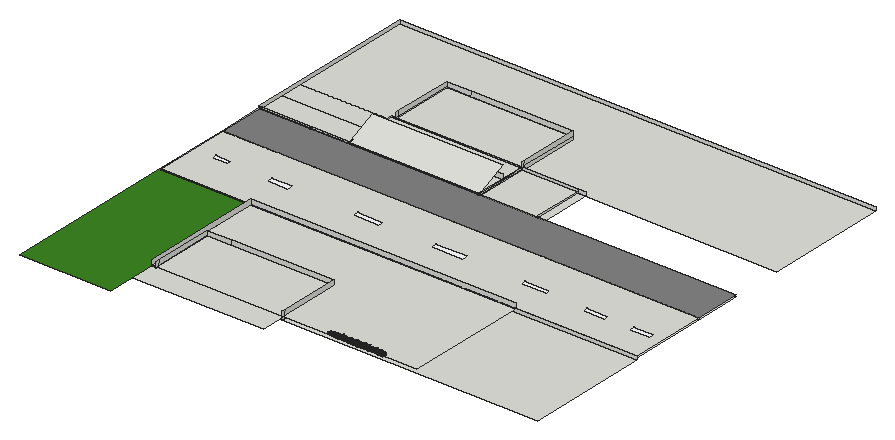
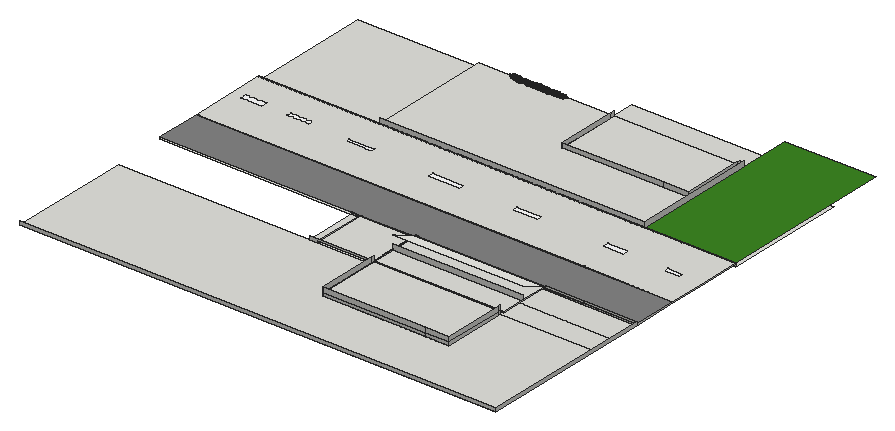
# SketchUp Ruby script. Lengths in inches.
U = 1.inch
M = Sketchup.active_model
def pt(a) = Geom::Point3d.new(a.map { |v| v * U })
def face(e, loops, mat)
  f = e.add_face(loops[0].map { |a| pt(a) })
  loops[1..].each { |l| e.add_face(l.map { |a| pt(a) }).erase! }
  f.material = f.back_material = mat if mat
  f
end
# faces: each face lists its corners as indices into pts; further lists are holes
def faces(e, pts, list, mat = nil) = list.each { |f| face(e, (f[0].is_a?(Array) ? f : [f]).map { |l| l.map { |i| pts[i] } }, mat) }
# xy, xz, yz: faces in a plane at the given z, y or x. An outline is a flat list of corners, or four numbers for a rectangle; further outlines are holes
def ring(l) = l.size == 4 ? [[l[0], l[1]], [l[2], l[1]], [l[2], l[3]], [l[0], l[3]]] : l.each_slice(2).to_a
def flat(e, list, mat, &to3) = list.each { |f| face(e, (f[0].is_a?(Array) ? f : [f]).map { |l| ring(l).map { |u, v| to3.(u, v) } }, mat) }
def xy(e, z, list, mat = nil) = flat(e, list, mat) { |x, y| [x, y, z] }
def xz(e, y, list, mat = nil) = flat(e, list, mat) { |x, z| [x, y, z] }
def yz(e, x, list, mat = nil) = flat(e, list, mat) { |y, z| [x, y, z] }
def lines(e, pts, list) = list.each { |a, b| e.add_line(pt(pts[a]), pt(pts[b])) }
# prism: a flat outline (further loops are holes) pulled along v
def prism(e, loops, v, mat = nil)
  f = face(e, loops, mat); d = Geom::Vector3d.new(v.map { |x| x * U })
  f.pushpull(f.normal.samedirection?(d) ? d.length : -d.length)
end
def box(e, o, s, mat = nil) = prism(e, [[o, [o[0] + s[0], o[1], o[2]], [o[0] + s[0], o[1] + s[1], o[2]], [o[0], o[1] + s[1], o[2]]]], [0, 0, s[2]], mat)
def at(x, y, z, deg = 0) = Geom::Transformation.translation(pt([x, y, z])) * Geom::Transformation.rotation(ORIGIN, Z_AXIS, deg.degrees)
def axes(o, x, y, z) = Geom::Transformation.new([*x, 0, *y, 0, *z, 0, *pt(o).to_a, 1])
def part(name) = M.definitions.add(name)
# library, detail: a bought-in or finely detailed component or shape, given as its bounding box
def library(name, o, s) = part(name).tap { |d| box(d.entities, o, s) }
def detail(e, o, s) = box(e.add_group.entities, o, s)
def put(e, d, t, mat = nil) = e.add_instance(d, t).tap { |i| i.material = mat if mat }
def group(e, t, mat = nil) = e.add_group.tap { |g| g.transformation = t; g.material = mat if mat }.entities
root = M.entities
M.materials.add("Color_3").color = [255, 255, 255]
M.materials.add("Material82").color = [68, 110, 58]
M.materials.add("Material83").color = [48, 90, 38]
M.materials.add("Material84").color = [68, 110, 48]
M.materials.add("Material85").color = [48, 90, 48]
M.materials.add("Material86").color = [58, 110, 58]
M.materials.add("Material87").color = [58, 90, 38]
M.materials.add("Material88").color = [68, 100, 58]
M.materials.add("Material89").color = [48, 100, 38]
M.materials.add("[Color M01]").color = [60, 133, 34]
M.materials.add("[Tile Grey]1").color = [132, 132, 132]
c1 = part("grass00")
p = [[-0.6875,0.15,0],[-0.56,0.08,5.52],[-0.04,0.03,2.76],[0.48,-0.02,0],[0.35,-0.02,5.52],[-0.1,-0.14,5.52],
  [-0.12,0.65,8.37],[-0.42,0.65,8.37]]
faces(c1.entities,p,[[0,1,2,3],[3,2,4],[1,5,2],[5,4,2],[1,6,5],[4,5,6],[7,6,1]])
c2 = part("Group16\#1")
put(c2.entities,c1,axes([1.44,-0.61,-0.01],[0.05352,0.12609,0],[-0.10704,0.04543,0.07239],[0.06664,-0.02828,0.11628]),"Material85")
put(c2.entities,c1,axes([0.76,-0.15,-0.01],[0.04676,0.24062,0],[-0.23162,0.04501,0.06642],[0.0652,-0.01267,0.23595]),"Material82")
put(c2.entities,c1,axes([0.79,0.01,-0.01],[-0.00606,0.34651,0],[-0.34381,-0.00602,0.0432],[0.04319,0.00076,0.34386]))
put(c2.entities,c1,axes([1,0.23,-0.01],[-0.07192,0.31144,0],[-0.28722,-0.06632,0.1236],[0.12043,0.02781,0.29478]),"Material84")
put(c2.entities,c1,axes([1.66,0.77,-0.01],[-0.13828,0.29651,0],[-0.21551,-0.1005,0.22471],[0.20365,0.09498,0.23779]),"Material89")
put(c2.entities,c1,axes([0.6875,0.52,-0.01],[-0.18126,0.24051,0],[-0.22746,-0.17142,0.09788],[0.07817,0.05891,0.28481]),"Material84")
put(c2.entities,c1,axes([0.68,0.78,-0.01],[-0.215,0.18688,0],[-0.12385,-0.14248,0.21334],[0.13995,0.16101,0.18878]),"Material82")
put(c2.entities,c1,axes([0.56,1,-0.01],[-0.13756,0.07624,0],[-0.06159,-0.11112,0.0927],[0.04494,0.08108,0.12705]),"Material84")
put(c2.entities,c1,axes([0.2,0.64,-0.01],[-0.23729,0.07254,0],[-0.05711,-0.18681,0.153],[0.04473,0.14632,0.19535]),"Material89")
put(c2.entities,c1,axes([0.0625,0.72,-0.01],[-0.28874,0.02525,0],[-0.02179,-0.24916,0.14647],[0.01276,0.14591,0.25012]),"Material82")
put(c2.entities,c1,axes([-0.08,0.62,-0.01],[-0.34089,-0.04187,0],[0.03255,-0.26504,0.216],[-0.02633,0.21439,0.26703]),"Material89")
put(c2.entities,c1,axes([-0.34,0.98,-0.01],[-0.14314,-0.0493,0],[0.04397,-0.12769,0.06843],[-0.02228,0.0647,0.13505]),"Material89")
put(c2.entities,c1,axes([-0.87,1.45,-0.01],[-0.23488,-0.14114,0],[0.13761,-0.22901,0.06087],[-0.03135,0.05217,0.26717]))
put(c2.entities,c1,axes([-0.72,0.77,-0.01],[-0.14208,-0.13251,0],[0.07209,-0.0773,0.16301],[-0.11118,0.11922,0.1057]),"Material89")
put(c2.entities,c1,axes([-0.62,0.43,-0.01],[-0.14845,-0.21203,0],[0.18654,-0.13061,0.12304],[-0.10079,0.07057,0.22772]),"Material82")
put(c2.entities,c1,axes([-0.68,0.29,-0.01],[-0.13639,-0.32136,0],[0.31723,-0.13464,0.05579],[-0.05136,0.0218,0.34462]),"Material83")
put(c2.entities,c1,axes([-0.64,0.125,-0.01],[-0.0458,-0.23569,0],[0.22124,-0.043,0.08276],[-0.08124,0.01579,0.22538]),"Material86")
put(c2.entities,c1,axes([-1.6,-0.03,-0.01],[0.00576,-0.32897,0],[0.27526,0.00482,0.18018],[-0.18015,-0.00315,0.2753]),"Material84")
put(c2.entities,c1,axes([-1.36,-0.31,-0.01],[0.05718,-0.24765,0],[0.18172,0.04196,0.17267],[-0.16825,-0.03885,0.1865]),"Material89")
put(c2.entities,c1,axes([-1.54,-0.72,-0.01],[0.06537,-0.14017,0],[0.13555,0.06321,0.03939],[-0.0357,-0.01665,0.14956]))
put(c2.entities,c1,axes([-1.19,-0.9,-0.01],[0.09597,-0.12735,0],[0.11214,0.08451,0.07557],[-0.06035,-0.04548,0.14042]),"Material88")
put(c2.entities,c1,axes([-0.47,-0.54,-0.01],[0.11588,-0.10072,0],[0.0618,0.0711,0.12124],[-0.07953,-0.0915,0.0942]))
put(c2.entities,c1,axes([-0.47,-0.84,-0.01],[0.11927,-0.0661,0],[0.06603,0.11913,0.00646],[-0.00313,-0.00565,0.13621]),"Material84")
put(c2.entities,c1,axes([-0.38,-1.24,-0.01],[0.28037,-0.08571,0],[0.0618,0.20215,0.20315],[-0.05939,-0.19428,0.21139]),"Material88")
put(c2.entities,c1,axes([-0.06,-0.66,-0.01],[0.22719,-0.01987,0],[0.01247,0.14255,0.17758],[-0.01547,-0.17691,0.1431]),"Material87")
put(c2.entities,c1,axes([0.11,-0.89,-0.01],[0.14882,0.01828,0],[-0.01058,0.08611,0.12229],[0.01491,-0.12138,0.08676]),"Material85")
put(c2.entities,c1,axes([0.25,-0.72,-0.01],[0.20481,0.07053,0],[-0.06206,0.18022,0.10291],[0.03351,-0.0973,0.1906]),"Material85")
put(c2.entities,c1,axes([0.85,-1.42,-0.01],[0.16481,0.09904,0],[-0.09472,0.15762,0.05616],[0.02893,-0.04814,0.18389]),"Material84")
put(c2.entities,c1,axes([1.01,-1.09,-0.01],[0.21858,0.20385,0],[-0.17495,0.1876,0.15339],[0.10462,-0.11218,0.25652]),"Material89")
put(c2.entities,c1,axes([1.01,-0.71,-0.01],[0.08733,0.12473,0],[-0.06445,0.04512,0.13037],[0.1068,-0.07477,0.07867]),"Material85")
c3 = part("Group15\#1")
put(c3.entities,c2,at(0,0,0))
c4 = part("3darcstudiotree_grass00\#1")
put(c4.entities,c3,at(0,0,0))
c5 = part("Untitled (5)")
xy(c5.entities,0,[[[158.81,26.5625,306.06,993.3125],[226.57,518.17,239.57,583.92],[225.28,357.51,237.28,411.51],[222.61,182.28,236.36,226.53],[239.71,931.55,251.46,972.3],[233.64,703.93,242.14,755.18],[240.05,835.03,248.8,880.53],[222.04,66.5,231.29,100.5]]])
xy(c5.entities,0,[[222.04,66.5,231.29,100.5],[222.61,182.28,236.36,226.53],[225.28,357.51,237.28,411.51],[226.57,518.17,239.57,583.92],[233.64,703.93,242.14,755.18],
  [240.05,835.03,248.8,880.53],[239.71,931.55,251.46,972.3]],"Color_3")
xy(root,-42.1875,[[0.34,387.84,0.34,659.09,1048.66,659.09,1048.66,387.84,486.41,387.84,486.41,528.53,208.91,528.53,208.91,387.84],[208.91,387.84,486.41,528.53]])
xy(root,-37.75,[[0,660.69,1048.3125,831.37],[0,831.37,199.6875,932.5],[199.6875,831.37,199.6875,932.5,486.07,932.5,486.07,1046.93,608.75,1046.93,608.75,932.5,1048.3125,932.5,1048.3125,831.37],[0,932.5,486.07,994.94],[608.75,932.5,626.34,1046.93],
  [0,994.94,486.07,1046.93],[0,1046.93,0,1318.18,1048.3125,1318.18,1048.3125,1046.93,486.07,1046.93,486.07,1187.62,208.57,1187.62,208.57,1046.93],[208.57,1046.93,486.07,1187.62]])
xy(root,-35.625,[[200.03,335.84,486.41,335.84,486.41,528.53,208.91,528.53,208.91,387.84,200.03,387.84]])
xy(root,-34.75,[[0,660.69,1048.3125,831.37]])
xy(root,-34.6875,[[486.07,932.5,608.75,1046.93]])
xy(root,-34.17,[[200.03,387.84,782.78,659.09]])
xy(root,-34.17,[[0.34,273.53,200.03,659.09]],"[Color M01]")
xy(root,-34.17,[[0,831.37,1048.3125,932.5]],"[Tile Grey]1")
xy(root,-33.625,[[0,932.5,115.625,932.62],[115.625,932.5,486.07,932.62]])
xy(root,-31.1875,[[199.6875,932.5,486.07,932.62],[199.6875,932.62,486.07,994.94],[199.6875,994.94,486.07,994.94,486.07,1187.62,208.57,1187.62,208.57,1046.93,199.6875,1046.93]])
xz(root,528.53,[[208.91,-42.1875,262.79,-35.625],[262.79,-42.1875,486.41,-35.625],[208.91,-35.625,262.79,-24.25],[262.79,-35.625,486.41,-24.25]])
xz(root,659.09,[[0.34,-42.1875,1048.66,-34.17],[200.03,-34.17,782.78,-22.8]])
xz(root,660.69,[[0,-37.75,1048.3125,-34.75]])
xz(root,831.37,[[0,-37.75,199.6875,-34.75],[199.6875,-37.75,1048.3125,-34.75],[0,-34.75,199.6875,-34.17],[199.6875,-34.75,1048.3125,-34.17]])
xz(root,932.5,[[0,-37.75,199.6875,-34.17],[199.6875,-37.75,486.07,-34.6875],[608.75,-37.75,626.34,-34.6875],[199.6875,-34.6875,486.07,-34.17],[486.07,-34.6875,608.75,-34.17],
  [608.75,-34.6875,626.34,-34.17],[0,-34.17,486.07,-33.75],[486.07,-34.17,608.75,-33.75],[608.75,-34.17,626.34,-33.75],[0,-33.75,486.07,-33.625],
  [115.625,-33.625,486.07,-33.625,486.07,-31.1875,199.6875,-31.1875,199.6875,-29.74,115.625,-29.74]])
xz(root,932.62,[[0,-33.625,115.625,-29.74],[115.625,-33.625,115.625,-29.74,199.6875,-29.74,199.6875,-31.1875,486.07,-31.1875,486.07,-33.625]])
xz(root,994.94,[[199.6875,-31.1875,486.07,-19.8125]])
xz(root,1046.93,[[208.57,-37.75,486.07,-29.74],[608.75,-37.75,626.34,-29.74],[486.07,-34.6875,608.75,-29.74],[199.6875,-31.1875,208.57,-29.74]])
xz(root,1187.62,[[208.57,-37.75,262.44,-31.1875],[262.44,-37.75,486.07,-31.1875],[208.57,-31.1875,262.44,-19.8125],[262.44,-31.1875,486.07,-19.8125]])
xz(root,1318.18,[[0,-37.75,1048.3125,-29.74]])
yz(root,0,[[660.69,-37.75,750.06,-34.75],[750.06,-37.75,831.37,-34.75],[831.37,-37.75,932.5,-34.17],[932.5,-37.75,932.5,-33.625,932.62,-33.625,932.62,-29.74,1318.18,-29.74,1318.18,-37.75]])
yz(root,115.625,[[932.5,-33.625,932.62,-29.74]])
yz(root,199.6875,[[932.5,-31.1875,932.62,-31.13,932.62,-29.74,932.5,-29.74],[932.5,-31.1875,932.62,-31.1875,932.62,-31.13],[932.62,-31.1875,932.62,-31.13,935.62,-29.74,994.94,-29.74,994.94,-31.1875],[994.94,-31.1875,1046.93,-29.74],[932.62,-31.13,935.62,-29.74,932.62,-29.74]])
yz(root,200.03,[[387.84,-34.17,659.09,-22.8]])
yz(root,208.57,[[1046.93,-37.75,1054,-31.1875],[1054,-37.75,1187.62,-31.1875],[1046.93,-31.1875,1054,-19.8125],[1054,-31.1875,1187.62,-19.8125]])
yz(root,208.91,[[387.84,-42.1875,394.91,-35.625],[394.91,-42.1875,528.53,-35.625],[387.84,-35.625,394.91,-24.25],[394.91,-35.625,528.53,-24.25]])
yz(root,486.07,[[932.5,-37.75,994.94,-34.6875],[994.94,-37.75,1022.06,-34.6875],[1022.06,-37.75,1023.55,-34.6875],[1023.55,-37.75,1046.93,-34.6875],[1046.93,-37.75,1054,-31.1875],
  [1054,-37.75,1187.62,-31.1875],[932.5,-34.6875,932.5,-33.625,932.62,-33.625,932.62,-31.1875,994.94,-31.1875,994.94,-34.6875],[994.94,-34.6875,1022.06,-31.1875],[1022.06,-34.6875,1023.55,-31.1875],[1023.55,-34.6875,1046.93,-31.1875],
  [932.5,-33.625,932.62,-33.42],[932.5,-33.42,932.62,-32.8],[932.5,-32.8,932.62,-31.1875],[932.5,-31.1875,932.5,-29.74,935.62,-29.74],[932.5,-31.1875,994.94,-31.1875,994.94,-29.74,935.62,-29.74],
  [994.94,-31.1875,1022.06,-29.74],[1022.06,-31.1875,1023.55,-29.74],[1023.55,-31.1875,1046.93,-29.74],[1046.93,-31.1875,1054,-19.8125],[1054,-31.1875,1187.62,-19.8125]])
yz(root,486.41,[[387.84,-42.1875,394.91,-35.625],[394.91,-42.1875,528.53,-35.625],[387.84,-35.625,394.91,-24.25],[394.91,-35.625,528.53,-24.25]])
yz(root,608.75,[[932.5,-37.75,1046.93,-34.6875]])
p = [[199.6875,994.94,-2.1875],[199.6875,935.62,-29.74],[199.6875,932.62,-31.13],[199.6875,932.5,-31.1875],[486.07,932.5,-31.1875],[486.07,935.62,-29.74],
  [486.07,994.94,-2.1875]]
faces(root,p,[[0,1,2,3,4,5,6]])
put(root,c4,axes([702.86,387.88,-34.17],[-2.85085,-0.66888,0],[2.41654,-1.60188,-0.00321],[0.00686,-0.00455,1.48019]))
put(root,c4,axes([609.45,388.31,-34.17],[3.43516,0.20919,0],[-0.57575,1.47043,-0.03647],[-0.03089,0.0789,1.56991]))
put(root,c4,axes([658.66,388.41,-34.17],[-3.1613,-1.38915,0],[3.20855,-1.13563,-0.02493],[0.08224,-0.02911,1.43253]))
put(root,c4,axes([679.95,388.5,-34.17],[-2.12705,-1.09895,0],[2.82257,-0.84968,-0.04177],[0.17079,-0.05141,1.36919]))
put(root,c4,axes([638.65,388.45,-34.17],[-3.25209,-0.85971,0],[2.35344,-1.3846,-0.05337],[0.14871,-0.08749,1.58535]))
put(root,c4,axes([705.02,388.16,-34.17],[-0.87127,1.65753,0],[-3.69619,-0.30217,-0.02464],[-0.15319,-0.01252,1.79662]))
put(root,c4,axes([653.34,388.66,-34.17],[-2.22741,-1.08823,0],[2.74712,-0.87452,-0.02577],[0.11865,-0.03777,1.56591]))
put(root,c4,axes([645.67,388.41,-34.17],[-3.60513,-0.15499,0],[0.46196,-1.67121,-0.01401],[0.00822,-0.02974,1.72979]))
put(root,c4,axes([656.98,389.55,-34.17],[2.77032,-1.11765,0],[2.79461,1.07735,-0.00015],[0.00071,0.00027,1.98495]))
put(root,c4,axes([653.21,389.375,-34.17],[-2.63384,-1.55649,0],[3.02127,-0.79514,-0.04802],[0.24921,-0.06559,1.69851]))
put(root,c4,axes([634.76,389.46,-34.17],[-0.69591,-1.28996,0],[3.84518,-0.32263,-0.04713],[0.24772,-0.02078,1.58351]))
put(root,c4,axes([648.09,389.5625,-34.17],[4.30833,-0.24109,0],[0.6166,1.71371,-0.05794],[0.04515,0.12549,1.82474]))
put(root,c4,axes([630.9,390.01,-34.17],[3.37733,-0.03199,0],[0.10215,1.67739,-0.04057],[0.00409,0.06713,1.33829]))
put(root,c4,axes([598.26,389.47,-34.17],[-2.59394,1.01102,0],[-3.072,-1.22583,-0.01852],[-0.05979,-0.02386,1.50457]))
put(root,c4,axes([616.88,390.41,-34.17],[2.33818,-1.41789,0],[2.84176,0.72884,-0.04791],[0.27889,0.07153,1.76421]))
put(root,c4,axes([622.5,390.47,-34.17],[0.86182,-1.33711,0],[3.4036,0.34119,-0.00558],[0.03445,0.00345,1.6757]))
put(root,c4,axes([702.69,390.18,-34.17],[2.4354,1.06288,0],[-2.86607,1.02137,-0.0306],[-0.14622,0.05211,1.86488]))
put(root,c4,axes([666.72,390.06,-34.17],[0.39811,1.50692,0],[-3.94981,0.16229,-0.02993],[-0.16157,0.00664,1.61572]))
put(root,c4,axes([689.78,390.23,-34.17],[-3.73597,-0.76469,0],[1.79369,-1.36294,-0.02416],[0.05526,-0.04199,1.4491]))
put(root,c4,axes([614.28,390.27,-34.17],[-3.25297,-0.61029,0],[1.91072,-1.58399,-0.03826],[0.09019,-0.07477,1.82966]))
put(root,c4,axes([662.96,390.8,-34.17],[3.60935,-0.56815,0],[1.37625,1.35979,-0.02611],[0.05001,0.04941,1.43783]))
put(root,c4,axes([603.89,390.22,-34.17],[-2.1063,1.53486,0],[-3.86767,-0.82549,-0.04902],[-0.23106,-0.04932,1.76654]))
put(root,c4,axes([694.69,390.64,-34.17],[-2.95598,-0.91326,0],[2.43781,-1.22721,-0.04081],[0.12436,-0.0626,1.46417]))
put(root,c4,axes([639.72,390.83,-34.17],[-3.50198,-0.71469,0],[1.86103,-1.41828,-0.02021],[0.05866,-0.0447,1.91641]))
put(root,c4,axes([679.9375,390.74,-34.17],[-0.65253,1.4678,0],[-3.82967,-0.26479,-0.02601],[-0.14603,-0.0101,1.66111]))
put(root,c4,axes([606.28,390.73,-34.17],[-1.7142,1.30326,0],[-3.68982,-0.75483,-0.04385],[-0.17675,-0.03616,1.41492]))
put(root,c4,axes([671.96,390.83,-34.17],[-4.08637,0.5893,0],[-1.1512,-1.24155,-0.04181],[-0.0785,-0.08466,1.37365]))
put(root,c4,axes([683.45,390.93,-34.17],[0.62564,1.8219,0],[-4.46763,0.23861,-0.03426],[-0.17796,0.0095,1.77113]))
put(root,c4,axes([614.12,391.67,-34.17],[2.39,-1.25303,0],[3.55352,1.05416,-0.05537],[0.20037,0.05944,1.50911]))
put(root,c4,axes([679.78,391.57,-34.17],[3.95759,-0.11816,0],[0.2883,1.50178,-0.04662],[0.02067,0.10765,1.68074]))
put(root,c4,axes([652.88,391.82,-34.17],[2.75838,0.79761,0],[-2.27657,1.22449,-0.01003],[-0.02813,0.01513,1.36834]))
put(root,c4,axes([701.06,392.06,-34.17],[0.25727,-1.4604,0],[3.98489,0.10918,-0.0172],[0.09613,0.00263,1.67763]))
put(root,c4,axes([646,391.5625,-34.17],[-1.99433,1.44629,0],[-3.30766,-0.70937,-0.03157],[-0.17706,-0.03797,1.80167]))
put(root,c4,axes([667.61,391.72,-34.17],[0.18137,1.61713,0],[-3.86456,0.06741,-0.03464],[-0.18684,0.00326,1.56527]))
put(root,c4,axes([641.48,392.26,-34.17],[3.4743,0.19553,0],[-0.61359,1.69568,-0.03434],[-0.02545,0.07034,1.70799]))
put(root,c4,axes([685.45,391.64,-34.17],[-2.17573,1.65884,0],[-3.97455,-0.81077,-0.04288],[-0.19169,-0.0391,1.68813]))
put(root,c4,axes([618.54,391.89,-34.17],[-1.73323,1.28831,0],[-3.70175,-0.77456,-0.05129],[-0.19346,-0.04048,1.34106]))
put(root,c4,axes([635.69,391.87,-34.17],[-4.09244,0.60833,0],[-1.31907,-1.38013,-0.00238],[-0.00395,-0.00413,1.31717]))
put(root,c4,axes([695.24,392.57,-34.17],[-0.4279,-1.35562,0],[4.45161,-0.21854,-0.05859],[0.31746,-0.01559,1.83593]))
put(root,c4,axes([674.92,392.16,-34.17],[-4.63629,0.17249,0],[-0.31305,-1.3087,-0.02738],[-0.01684,-0.0704,1.63584]))
put(root,c4,axes([609.39,392.67,-34.17],[-1.23898,-1.77649,0],[4.18164,-0.45359,-0.02011],[0.11729,-0.01272,1.9663]))
put(root,c4,axes([658.41,392.46,-34.17],[-4.11217,-0.39094,0],[0.86082,-1.40827,-0.01967],[0.02693,-0.04406,1.60841]))
put(root,c4,axes([689.19,392.9375,-34.17],[3.58477,-0.09461,0],[0.24683,1.45461,-0.02393],[0.00869,0.05119,1.50627]))
put(root,c4,axes([602.05,392.72,-34.17],[-2.67553,-0.98375,0],[2.79136,-1.18074,-0.04642],[0.15585,-0.06593,1.51042]))
put(root,c4,axes([597.59,392.39,-34.17],[-1.47744,1.354,0],[-3.50661,-0.5951,-0.01574],[-0.08407,-0.01427,1.66349]))
put(root,c4,axes([661.55,392.99,-34.17],[-0.90047,-1.75818,0],[4.05941,-0.32336,-0.03802],[0.21461,-0.0171,1.78771]))
put(root,c4,axes([622.83,392.71,-34.17],[-1.19077,1.57344,0],[-3.27951,-0.38601,-0.00408],[-0.02113,-0.00249,1.38631]))
put(root,c4,axes([629.5,392.99,-34.17],[1.23256,1.36805,0],[-3.36714,0.47182,-0.0026],[-0.01342,0.00188,1.46428]))
put(root,c4,axes([667.38,393.86,-34.17],[2.68425,0.98126,0],[-3.08103,1.31083,-0.0132],[-0.04194,0.01784,1.58767]))
put(root,c4,axes([639.33,394.0625,-34.17],[2.94498,0.60485,0],[-2.04543,1.54892,-0.0178],[-0.03241,0.02454,1.30843]))
put(root,c4,axes([611.83,393.84,-34.17],[-3.78694,0.18795,0],[-0.43899,-1.37568,-0.01354],[-0.00909,-0.02849,1.41676]))
put(root,c4,axes([686.49,394.19,-34.17],[1.29207,1.70529,0],[-3.1938,0.37636,-0.01522],[-0.08109,0.00956,1.38916]))
put(root,c4,axes([624.62,394.45,-34.17],[-2.41696,-1.08887,0],[3.39352,-1.17154,-0.03006],[0.11594,-0.04003,1.73276]))
put(root,c4,axes([660.98,394.24,-34.17],[-3.99047,-0.40873,0],[1.06863,-1.62266,-0.00758],[0.01027,-0.0156,1.7185]))
put(root,c4,axes([650.76,394.29,-34.17],[-4.3017,0.59676,0],[-1.104,-1.2377,-0.00518],[-0.01285,-0.0144,1.86492]))
put(root,c5,axes([-28.47,1017.18,-34.17],[0,-1.17,0],[1.0847,0,0],[0,0,1]))
